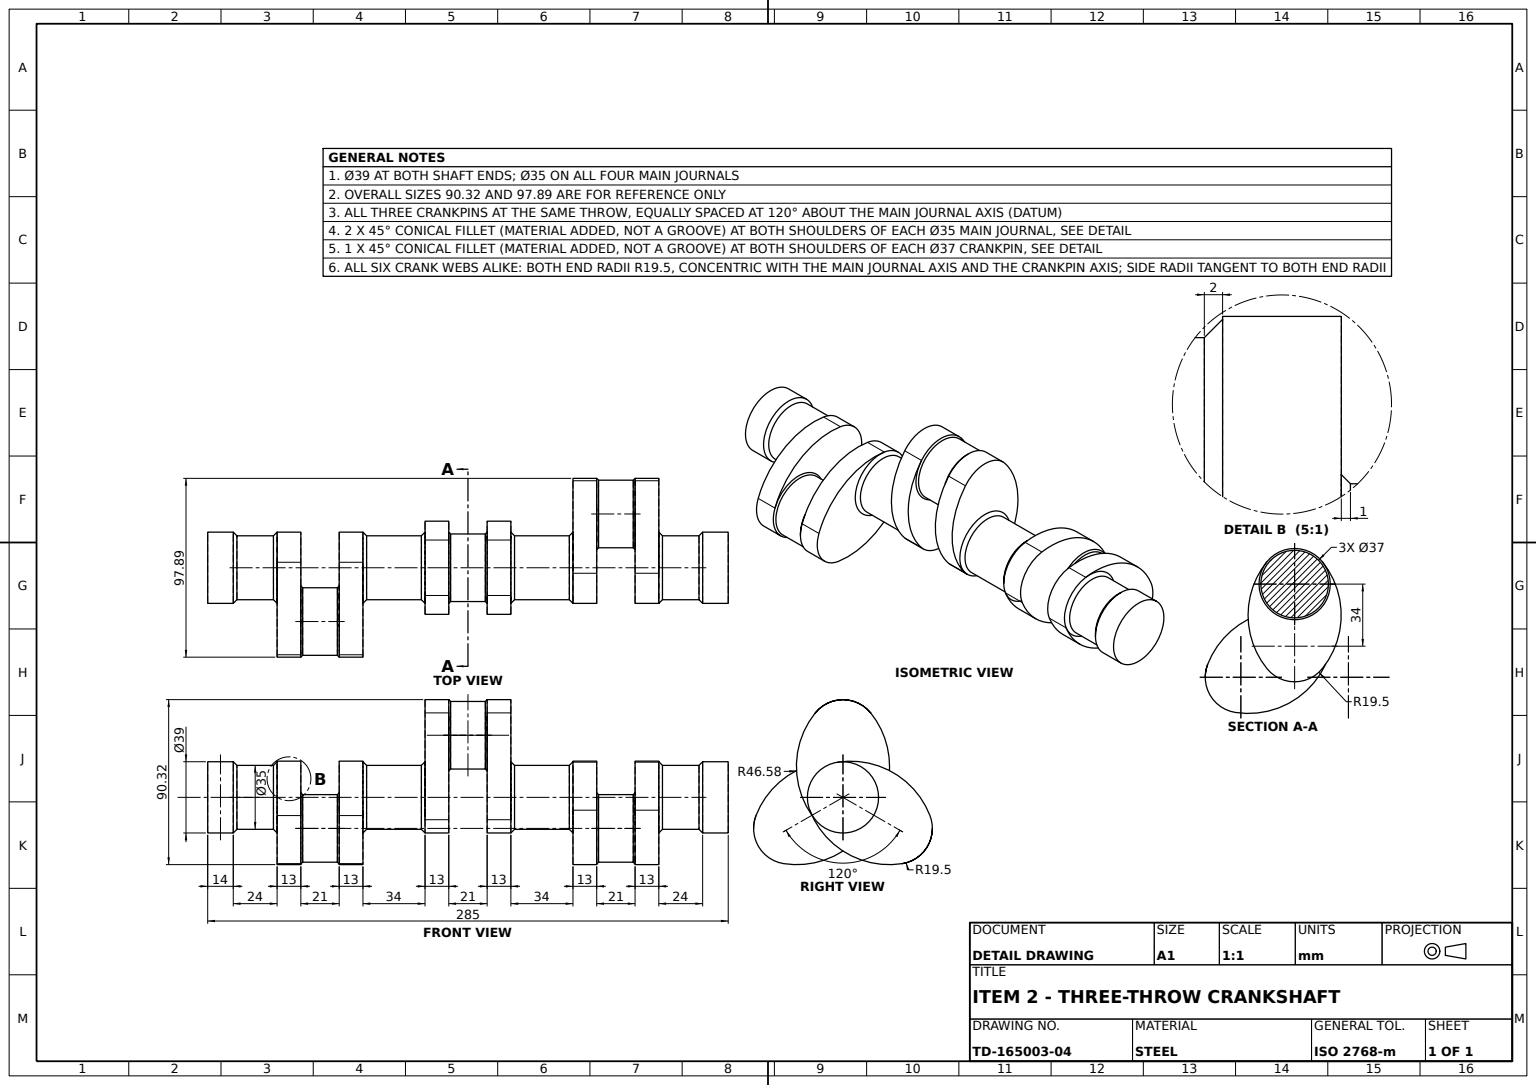
solid
v1 (247,0,19.5)
v2 (233,0,19.5)
e1 v1 v2 LINE
v3 (233,0,-19.5)
e2 v2 v3 CIRCLE(AX(P(233,0,0),D(1,0,0),D(0,0,-1)),19.5)
v4 (247,0,-19.5)
e3 v4 v3 LINE
e4 v1 v4 CIRCLE(AX(P(247,0,0),D(1,0,0),D(0,0,-1)),19.5)
face CYL(AX(P(247,0,0),D(-1,0,0),D(0,0,1)),19.5) [e1 e2 -e3 -e4]
v5 (196,-17,-9.9448637287)
v6 (196,-36.2662656294,-32.455014671)
e5 v5 v6 CIRCLE(AX(P(196,-17,-29.4448637287),D(1,0,0),D(0,0,1)),19.5)
v7 (196,-7.0262656294,18.1901509423)
e6 v7 v6 CIRCLE(AX(P(196,9.7587022631,-25.264098531),D(1,0,0),D(0,0,-1)),46.5833333333)
v8 (196,19.2662656294,3.0101509423)
e7 v8 v7 CIRCLE(AX(P(196,0,0),D(1,0,0),D(0,0,-1)),19.5)
v9 (196,-9.9737343706,-47.635014671)
e8 v9 v8 CIRCLE(AX(P(196,-26.7587022631,-4.1807651977),D(1,0,0),D(0,0,-1)),46.5833333333)
e9 v9 v5 CIRCLE(AX(P(196,-17,-29.4448637287),D(1,0,0),D(0,0,1)),19.5)
face PLANE(AX(P(196,-13.3793511316,-2.0903825988),D(-1,0,0),D(0,0,-1))) [e5 -e6 -e7 -e8 e9]
v10 (231,0,17.5)
e10 v10 v2 LINE
v11 (231,0,-17.5)
e11 v11 v10 CIRCLE(AX(P(231,0,0),D(-1,0,0),D(0,0,-1)),17.5)
e12 v11 v3 LINE
face CONE(AX(P(233,0,0),D(1,0,0),D(0,0,-1)),19.5,0.7853981634) [-e10 -e11 e12 -e2]
v12 (0,-9.9737343706,47.635014671)
v13 (0,-17,48.9448637287)
e13 v12 v13 CIRCLE(AX(P(0,-17,29.4448637287),D(1,0,0),D(0,0,-1)),19.5)
v14 (13,-17,48.9448637287)
e14 v14 v13 LINE
v15 (13,-9.9737343706,47.635014671)
e15 v15 v14 CIRCLE(AX(P(13,-17,29.4448637287),D(1,0,0),D(0,0,-1)),19.5)
e16 v15 v12 LINE
face CYL(AX(P(13,-17,29.4448637287),D(-1,0,0),D(0,0,1)),19.5) [e13 -e14 -e15 e16]
v16 (-38,0,19.5)
v17 (-38,0,-19.5)
e17 v16 v17 CIRCLE(AX(P(-38,0,0),D(1,0,0),D(0,0,-1)),19.5)
e18 v17 v16 CIRCLE(AX(P(-38,0,0),D(1,0,0),D(0,0,-1)),19.5)
face PLANE(AX(P(-38,19.5,0),D(-1,0,0),D(0,0,1))) [-e17 -e18]
v18 (-2,0,-17.5)
v19 (-2,0,17.5)
e19 v18 v19 CIRCLE(AX(P(-2,0,0),D(-1,0,0),D(0,0,1)),17.5)
v20 (0,0,-19.5)
e20 v18 v20 LINE
v21 (0,-7.0262656294,-18.1901509423)
e21 v21 v20 CIRCLE(AX(P(0,0,0),D(1,0,0),D(0,0,-1)),19.5)
v22 (0,0,19.5)
e22 v22 v21 CIRCLE(AX(P(0,0,0),D(1,0,0),D(0,0,1)),19.5)
e23 v19 v22 LINE
face CONE(AX(P(0,0,0),D(1,0,0),D(0,0,-1)),19.5,0.7853981634) [-e19 e20 -e21 -e22 -e23]
e24 v4 v1 CIRCLE(AX(P(247,0,0),D(1,0,0),D(0,0,-1)),19.5)
face PLANE(AX(P(247,0,0),D(1,0,0),D(0,0,-1))) [e24 e4]
v23 (128,-12.24,15.18)
v24 (128,-12.24,-15.18)
e25 v23 v24 CIRCLE(AX(P(128,0,0),D(1,0,0),D(0,0,-1)),19.5)
v25 (115,-12.24,15.18)
e26 v25 v23 LINE
v26 (115,-12.24,-15.18)
e27 v25 v26 CIRCLE(AX(P(115,0,0),D(1,0,0),D(0,0,-1)),19.5)
e28 v26 v24 LINE
face CYL(AX(P(115,0,0),D(1,0,0),D(0,0,-1)),19.5) [-e25 -e26 e27 e28]
v27 (114,34,18.5)
v28 (95,34,18.5)
e29 v27 v28 LINE
v29 (114,34,-18.5)
e30 v27 v29 CIRCLE(AX(P(114,34,0),D(-1,0,0),D(0,0,1)),18.5)
v30 (95,34,-18.5)
e31 v29 v30 LINE
e32 v30 v28 CIRCLE(AX(P(95,34,0),D(1,0,0),D(0,0,-1)),18.5)
face CYL(AX(P(115,34,0),D(-1,0,0),D(0,0,1)),18.5) [-e29 e30 e31 e32]
v31 (128,46.24,15.18)
e33 v31 v23 CIRCLE(AX(P(128,17,-21.0833333333),D(1,0,0),D(0,0,-1)),46.5833333333)
v32 (115,46.24,15.18)
e34 v32 v31 LINE
e35 v32 v25 CIRCLE(AX(P(115,17,-21.0833333333),D(1,0,0),D(0,0,-1)),46.5833333333)
face CYL(AX(P(115,17,-21.0833333333),D(1,0,0),D(0,0,-1)),46.5833333333) [e26 -e33 -e34 e35]
v33 (160,0,-17.5)
v34 (162,0,-19.5)
e36 v33 v34 LINE
v35 (162,-7.0262656294,18.1901509423)
e37 v35 v34 CIRCLE(AX(P(162,0,0),D(1,0,0),D(0,0,-1)),19.5)
v36 (162,0,19.5)
e38 v36 v35 CIRCLE(AX(P(162,0,0),D(1,0,0),D(0,0,-1)),19.5)
v37 (160,0,17.5)
e39 v37 v36 LINE
e40 v33 v37 CIRCLE(AX(P(160,0,0),D(-1,0,0),D(0,0,-1)),17.5)
face CONE(AX(P(162,0,0),D(1,0,0),D(0,0,-1)),19.5,0.7853981634) [e36 -e37 -e38 -e39 -e40]
v38 (49,0,-17.5)
v39 (49,0,17.5)
e41 v38 v39 CIRCLE(AX(P(49,0,0),D(1,0,0),D(0,0,-1)),17.5)
v40 (47,0,-19.5)
e42 v38 v40 LINE
v41 (47,19.2662656294,-3.0101509423)
e43 v40 v41 CIRCLE(AX(P(47,0,0),D(1,0,0),D(0,0,-1)),19.5)
v42 (47,0,19.5)
e44 v42 v41 CIRCLE(AX(P(47,0,0),D(-1,0,0),D(0,0,-1)),19.5)
e45 v39 v42 LINE
face CONE(AX(P(49,0,0),D(-1,0,0),D(0,0,1)),17.5,0.7853981634) [-e41 e42 e43 -e44 -e45]
v43 (195,-17,-47.9448637287)
v44 (176,-17,-47.9448637287)
e46 v43 v44 LINE
v45 (176,-17,-10.9448637287)
e47 v44 v45 CIRCLE(AX(P(176,-17,-29.4448637287),D(1,0,0),D(0,0,-1)),18.5)
v46 (195,-17,-10.9448637287)
e48 v46 v45 LINE
e49 v46 v43 CIRCLE(AX(P(195,-17,-29.4448637287),D(-1,0,0),D(0,0,1)),18.5)
face CYL(AX(P(196,-17,-29.4448637287),D(-1,0,0),D(0,0,1)),18.5) [e46 e47 -e48 e49]
e50 v37 v33 CIRCLE(AX(P(160,0,0),D(-1,0,0),D(0,0,-1)),17.5)
v47 (130,0,-17.5)
e51 v33 v47 LINE
v48 (130,0,17.5)
e52 v47 v48 CIRCLE(AX(P(130,0,0),D(1,0,0),D(0,0,1)),17.5)
e53 v37 v48 LINE
face CYL(AX(P(162,0,0),D(-1,0,0),D(0,0,1)),17.5) [e50 e51 e52 -e53]
v49 (33,-17,10.9448637287)
v50 (33,-17,47.9448637287)
e54 v49 v50 CIRCLE(AX(P(33,-17,29.4448637287),D(-1,0,0),D(0,0,-1)),18.5)
v51 (34,-17,9.9448637287)
e55 v49 v51 LINE
v52 (34,-36.2662656294,32.455014671)
e56 v52 v51 CIRCLE(AX(P(34,-17,29.4448637287),D(1,0,0),D(0,0,-1)),19.5)
v53 (34,-17,48.9448637287)
e57 v53 v52 CIRCLE(AX(P(34,-17,29.4448637287),D(1,0,0),D(0,0,-1)),19.5)
e58 v50 v53 LINE
face CONE(AX(P(34,-17,29.4448637287),D(1,0,0),D(0,0,-1)),19.5,0.7853981634) [-e54 e55 -e56 -e57 -e58]
v54 (94,46.24,-15.18)
v55 (94,46.24,15.18)
e59 v54 v55 CIRCLE(AX(P(94,34,0),D(1,0,0),D(0,0,-1)),19.5)
v56 (81,46.24,-15.18)
e60 v54 v56 LINE
v57 (81,46.24,15.18)
e61 v56 v57 CIRCLE(AX(P(81,34,0),D(1,0,0),D(0,0,-1)),19.5)
e62 v55 v57 LINE
face CYL(AX(P(94,34,0),D(-1,0,0),D(0,0,1)),19.5) [-e59 e60 e61 -e62]
e63 v10 v11 CIRCLE(AX(P(231,0,0),D(-1,0,0),D(0,0,-1)),17.5)
v58 (211,0,-17.5)
e64 v11 v58 LINE
v59 (211,0,17.5)
e65 v58 v59 CIRCLE(AX(P(211,0,0),D(1,0,0),D(0,0,1)),17.5)
e66 v10 v59 LINE
face CYL(AX(P(233,0,0),D(-1,0,0),D(0,0,1)),17.5) [e63 e64 e65 -e66]
v60 (34,-9.9737343706,47.635014671)
v61 (47,-9.9737343706,47.635014671)
e67 v60 v61 LINE
e68 v60 v53 CIRCLE(AX(P(34,-17,29.4448637287),D(1,0,0),D(0,0,-1)),19.5)
v62 (47,-36.2662656294,32.455014671)
e69 v52 v62 LINE
e70 v61 v62 CIRCLE(AX(P(47,-17,29.4448637287),D(1,0,0),D(0,0,-1)),19.5)
face CYL(AX(P(34,-17,29.4448637287),D(1,0,0),D(0,0,-1)),19.5) [-e67 e68 e57 e69 -e70]
e71 v29 v27 CIRCLE(AX(P(114,34,0),D(-1,0,0),D(0,0,1)),18.5)
e72 v28 v30 CIRCLE(AX(P(95,34,0),D(1,0,0),D(0,0,-1)),18.5)
face CYL(AX(P(115,34,0),D(-1,0,0),D(0,0,1)),18.5) [-e31 e71 e29 e72]
e73 v39 v38 CIRCLE(AX(P(49,0,0),D(1,0,0),D(0,0,-1)),17.5)
v63 (47,-7.0262656294,-18.1901509423)
e74 v63 v42 CIRCLE(AX(P(47,0,0),D(-1,0,0),D(0,0,-1)),19.5)
e75 v63 v40 CIRCLE(AX(P(47,0,0),D(1,0,0),D(0,0,-1)),19.5)
face CONE(AX(P(49,0,0),D(-1,0,0),D(0,0,1)),17.5,0.7853981634) [-e73 e45 -e74 e75 -e42]
v64 (13,-17,9.9448637287)
e76 v15 v64 CIRCLE(AX(P(13,-17,29.4448637287),D(-1,0,0),D(0,0,1)),19.5)
v65 (13,-36.2662656294,32.455014671)
e77 v64 v65 CIRCLE(AX(P(13,-17,29.4448637287),D(-1,0,0),D(0,0,1)),19.5)
v66 (13,-7.0262656294,-18.1901509423)
e78 v65 v66 CIRCLE(AX(P(13,9.7587022631,25.264098531),D(1,0,0),D(0,0,-1)),46.5833333333)
v67 (13,19.2662656294,-3.0101509423)
e79 v66 v67 CIRCLE(AX(P(13,0,0),D(1,0,0),D(0,0,-1)),19.5)
e80 v67 v15 CIRCLE(AX(P(13,-26.7587022631,4.1807651977),D(1,0,0),D(0,0,1)),46.5833333333)
face PLANE(AX(P(13,-13.3793511316,2.0903825988),D(-1,0,0),D(0,0,1))) rev [e76 e77 e78 e79 e80]
e81 v43 v46 CIRCLE(AX(P(195,-17,-29.4448637287),D(-1,0,0),D(0,0,1)),18.5)
e82 v45 v44 CIRCLE(AX(P(176,-17,-29.4448637287),D(1,0,0),D(0,0,-1)),18.5)
face CYL(AX(P(196,-17,-29.4448637287),D(-1,0,0),D(0,0,1)),18.5) [-e46 e81 e48 e82]
v68 (175,-9.9737343706,-47.635014671)
v69 (162,-9.9737343706,-47.635014671)
e83 v68 v69 LINE
v70 (175,-17,-48.9448637287)
e84 v70 v68 CIRCLE(AX(P(175,-17,-29.4448637287),D(1,0,0),D(0,0,-1)),19.5)
v71 (175,-36.2662656294,-32.455014671)
e85 v71 v70 CIRCLE(AX(P(175,-17,-29.4448637287),D(1,0,0),D(0,0,-1)),19.5)
v72 (162,-36.2662656294,-32.455014671)
e86 v71 v72 LINE
e87 v72 v69 CIRCLE(AX(P(162,-17,-29.4448637287),D(1,0,0),D(0,0,-1)),19.5)
face CYL(AX(P(175,-17,-29.4448637287),D(-1,0,0),D(0,0,1)),19.5) [-e83 -e84 -e85 e86 e87]
v73 (-24,0,-19.5)
e88 v17 v73 LINE
v74 (-24,0,19.5)
e89 v16 v74 LINE
e90 v73 v74 CIRCLE(AX(P(-24,0,0),D(1,0,0),D(0,0,-1)),19.5)
face CYL(AX(P(0,0,0),D(1,0,0),D(0,0,-1)),19.5) [-e88 e18 e89 -e90]
v75 (128,0,-19.5)
e91 v75 v24 CIRCLE(AX(P(128,0,0),D(-1,0,0),D(0,0,1)),19.5)
e92 v47 v75 LINE
e93 v48 v47 CIRCLE(AX(P(130,0,0),D(1,0,0),D(0,0,1)),17.5)
v76 (128,0,19.5)
e94 v48 v76 LINE
e95 v23 v76 CIRCLE(AX(P(128,0,0),D(-1,0,0),D(0,0,1)),19.5)
face CONE(AX(P(130,0,0),D(-1,0,0),D(0,0,1)),17.5,0.7853981634) [-e91 -e92 -e93 e94 -e95 e25]
e96 v3 v2 CIRCLE(AX(P(233,0,0),D(1,0,0),D(0,0,-1)),19.5)
face CYL(AX(P(247,0,0),D(-1,0,0),D(0,0,1)),19.5) [-e1 -e24 e3 e96]
v77 (79,0,-17.5)
e97 v77 v38 LINE
v78 (79,0,17.5)
e98 v78 v39 LINE
e99 v78 v77 CIRCLE(AX(P(79,0,0),D(-1,0,0),D(0,0,-1)),17.5)
face CYL(AX(P(81,0,0),D(-1,0,0),D(0,0,1)),17.5) [e97 e41 -e98 e99]
v79 (196,-17,-48.9448637287)
e100 v79 v9 CIRCLE(AX(P(196,-17,-29.4448637287),D(1,0,0),D(0,0,-1)),19.5)
e101 v43 v79 LINE
e102 v46 v5 LINE
face CONE(AX(P(196,-17,-29.4448637287),D(1,0,0),D(0,0,-1)),19.5,0.7853981634) [-e9 -e100 -e101 -e49 e102]
v80 (-22,0,17.5)
v81 (-22,0,-17.5)
e103 v80 v81 CIRCLE(AX(P(-22,0,0),D(1,0,0),D(0,0,-1)),17.5)
e104 v81 v18 LINE
e105 v80 v19 LINE
face CYL(AX(P(0,0,0),D(1,0,0),D(0,0,-1)),17.5) [e103 e104 e19 -e105]
v82 (162,19.2662656294,3.0101509423)
e106 v34 v82 CIRCLE(AX(P(162,0,0),D(1,0,0),D(0,0,-1)),19.5)
e107 v82 v36 CIRCLE(AX(P(162,0,0),D(1,0,0),D(0,0,-1)),19.5)
face CONE(AX(P(162,0,0),D(1,0,0),D(0,0,-1)),19.5,0.7853981634) [-e106 -e36 -e50 e39 -e107]
e108 v41 v61 CIRCLE(AX(P(47,-26.7587022631,4.1807651977),D(1,0,0),D(0,0,1)),46.5833333333)
e109 v62 v63 CIRCLE(AX(P(47,9.7587022631,25.264098531),D(1,0,0),D(0,0,-1)),46.5833333333)
face PLANE(AX(P(47,-13.3793511316,2.0903825988),D(1,0,0),D(0,0,1))) [e74 e44 e108 e70 e109]
e110 v59 v58 CIRCLE(AX(P(211,0,0),D(1,0,0),D(0,0,1)),17.5)
face CYL(AX(P(233,0,0),D(-1,0,0),D(0,0,1)),17.5) [-e64 e11 e66 e110]
e111 v80 v74 LINE
e112 v81 v80 CIRCLE(AX(P(-22,0,0),D(1,0,0),D(0,0,-1)),17.5)
e113 v81 v73 LINE
face CONE(AX(P(-22,0,0),D(-1,0,0),D(0,0,1)),17.5,0.7853981634) [e90 -e111 -e112 e113]
e114 v6 v79 CIRCLE(AX(P(196,-17,-29.4448637287),D(1,0,0),D(0,0,-1)),19.5)
face CONE(AX(P(196,-17,-29.4448637287),D(1,0,0),D(0,0,-1)),19.5,0.7853981634) [e101 -e114 -e5 -e102 -e81]
v83 (34,-7.0262656294,-18.1901509423)
e115 v83 v63 LINE
v84 (34,0,-19.5)
e116 v83 v84 CIRCLE(AX(P(34,0,0),D(1,0,0),D(0,0,-1)),19.5)
e117 v84 v40 LINE
face CYL(AX(P(34,0,0),D(1,0,0),D(0,0,-1)),19.5) [-e75 -e115 e116 e117]
v85 (81,0,19.5)
e118 v78 v85 LINE
v86 (81,0,-19.5)
e119 v86 v85 CIRCLE(AX(P(81,0,0),D(1,0,0),D(0,0,-1)),19.5)
e120 v77 v86 LINE
face CONE(AX(P(81,0,0),D(1,0,0),D(0,0,-1)),19.5,0.7853981634) [e118 -e119 -e120 -e99]
v87 (94,34,-19.5)
v88 (94,34,19.5)
e121 v87 v88 CIRCLE(AX(P(94,34,0),D(-1,0,0),D(0,0,-1)),19.5)
e122 v30 v87 LINE
e123 v28 v88 LINE
face CONE(AX(P(95,34,0),D(-1,0,0),D(0,0,1)),18.5,0.7853981634) [-e121 -e122 -e72 e123]
v89 (94,-12.24,15.18)
v90 (94,-12.24,-15.18)
e124 v89 v90 CIRCLE(AX(P(94,0,0),D(1,0,0),D(0,0,-1)),19.5)
v91 (81,-12.24,15.18)
e125 v89 v91 LINE
v92 (81,-12.24,-15.18)
e126 v91 v92 CIRCLE(AX(P(81,0,0),D(1,0,0),D(0,0,-1)),19.5)
e127 v90 v92 LINE
face CYL(AX(P(94,0,0),D(-1,0,0),D(0,0,1)),19.5) [-e124 e125 e126 -e127]
v93 (209,-7.0262656294,18.1901509423)
v94 (209,-36.2662656294,-32.455014671)
e128 v93 v94 CIRCLE(AX(P(209,9.7587022631,-25.264098531),D(1,0,0),D(0,0,-1)),46.5833333333)
v95 (209,-17,-48.9448637287)
e129 v94 v95 CIRCLE(AX(P(209,-17,-29.4448637287),D(1,0,0),D(0,0,-1)),19.5)
v96 (209,-9.9737343706,-47.635014671)
e130 v95 v96 CIRCLE(AX(P(209,-17,-29.4448637287),D(1,0,0),D(0,0,-1)),19.5)
v97 (209,19.2662656294,3.0101509423)
e131 v96 v97 CIRCLE(AX(P(209,-26.7587022631,-4.1807651977),D(1,0,0),D(0,0,-1)),46.5833333333)
v98 (209,0,-19.5)
e132 v97 v98 CIRCLE(AX(P(209,0,0),D(-1,0,0),D(0,0,1)),19.5)
e133 v98 v93 CIRCLE(AX(P(209,0,0),D(-1,0,0),D(0,0,1)),19.5)
face PLANE(AX(P(209,-13.3793511316,-2.0903825988),D(-1,0,0),D(0,0,-1))) rev [e128 e129 e130 e131 e132 e133]
v99 (0,-36.2662656294,32.455014671)
e134 v13 v99 CIRCLE(AX(P(0,-17,29.4448637287),D(1,0,0),D(0,0,-1)),19.5)
v100 (0,19.2662656294,-3.0101509423)
e135 v100 v12 CIRCLE(AX(P(0,-26.7587022631,4.1807651977),D(1,0,0),D(0,0,1)),46.5833333333)
e136 v100 v22 CIRCLE(AX(P(0,0,0),D(1,0,0),D(0,0,1)),19.5)
e137 v99 v21 CIRCLE(AX(P(0,9.7587022631,25.264098531),D(1,0,0),D(0,0,-1)),46.5833333333)
face PLANE(AX(P(0,-13.3793511316,2.0903825988),D(-1,0,0),D(0,0,1))) [-e134 -e13 -e135 e136 e22 -e137]
face CONE(AX(P(233,0,0),D(1,0,0),D(0,0,-1)),19.5,0.7853981634) [-e12 -e63 e10 -e96]
e138 v92 v56 CIRCLE(AX(P(81,17,21.0833333333),D(1,0,0),D(0,0,-1)),46.5833333333)
e139 v90 v54 CIRCLE(AX(P(94,17,21.0833333333),D(1,0,0),D(0,0,-1)),46.5833333333)
face CYL(AX(P(94,17,21.0833333333),D(-1,0,0),D(0,0,1)),46.5833333333) [e127 e138 -e60 -e139]
e140 v67 v100 LINE
face CYL(AX(P(13,-26.7587022631,4.1807651977),D(-1,0,0),D(0,0,1)),46.5833333333) [e135 -e16 -e80 e140]
e141 v9 v96 LINE
e142 v8 v97 LINE
face CYL(AX(P(196,-26.7587022631,-4.1807651977),D(1,0,0),D(0,0,-1)),46.5833333333) [-e131 -e141 e8 e142]
v101 (209,0,19.5)
e143 v101 v93 CIRCLE(AX(P(209,0,0),D(1,0,0),D(0,0,-1)),19.5)
e144 v58 v98 LINE
e145 v59 v101 LINE
face CONE(AX(P(211,0,0),D(-1,0,0),D(0,0,1)),17.5,0.7853981634) [e143 -e133 -e144 -e110 e145]
e146 v52 v83 CIRCLE(AX(P(34,9.7587022631,25.264098531),D(1,0,0),D(0,0,-1)),46.5833333333)
face CYL(AX(P(34,9.7587022631,25.264098531),D(1,0,0),D(0,0,-1)),46.5833333333) [e115 -e109 -e69 e146]
e147 v74 v73 CIRCLE(AX(P(-24,0,0),D(1,0,0),D(0,0,-1)),19.5)
face CONE(AX(P(-22,0,0),D(-1,0,0),D(0,0,1)),17.5,0.7853981634) [-e103 e111 e147 -e113]
v102 (115,34,-19.5)
e148 v29 v102 LINE
v103 (115,34,19.5)
e149 v103 v102 CIRCLE(AX(P(115,34,0),D(1,0,0),D(0,0,1)),19.5)
e150 v27 v103 LINE
face CONE(AX(P(115,34,0),D(1,0,0),D(0,0,-1)),19.5,0.7853981634) [-e71 e148 -e149 -e150]
e151 v97 v101 CIRCLE(AX(P(209,0,0),D(1,0,0),D(0,0,-1)),19.5)
face CONE(AX(P(211,0,0),D(-1,0,0),D(0,0,1)),17.5,0.7853981634) [e144 -e132 e151 -e145 -e65]
v104 (175,19.2662656294,3.0101509423)
e152 v68 v104 CIRCLE(AX(P(175,-26.7587022631,-4.1807651977),D(1,0,0),D(0,0,-1)),46.5833333333)
e153 v69 v82 CIRCLE(AX(P(162,-26.7587022631,-4.1807651977),D(1,0,0),D(0,0,-1)),46.5833333333)
e154 v104 v82 LINE
face CYL(AX(P(175,-26.7587022631,-4.1807651977),D(-1,0,0),D(0,0,1)),46.5833333333) [-e152 e83 e153 -e154]
e155 v92 v86 CIRCLE(AX(P(81,0,0),D(1,0,0),D(0,0,-1)),19.5)
e156 v85 v91 CIRCLE(AX(P(81,0,0),D(1,0,0),D(0,0,-1)),19.5)
e157 v77 v78 CIRCLE(AX(P(79,0,0),D(-1,0,0),D(0,0,-1)),17.5)
face CONE(AX(P(81,0,0),D(1,0,0),D(0,0,-1)),19.5,0.7853981634) [e120 -e155 -e126 -e156 -e118 -e157]
e158 v6 v94 LINE
e159 v7 v93 LINE
face CYL(AX(P(196,9.7587022631,-25.264098531),D(1,0,0),D(0,0,-1)),46.5833333333) [e6 e158 -e128 -e159]
v105 (14,-17,10.9448637287)
e160 v49 v105 LINE
v106 (14,-17,47.9448637287)
e161 v105 v106 CIRCLE(AX(P(14,-17,29.4448637287),D(1,0,0),D(0,0,1)),18.5)
e162 v50 v106 LINE
e163 v50 v49 CIRCLE(AX(P(33,-17,29.4448637287),D(-1,0,0),D(0,0,-1)),18.5)
face CYL(AX(P(34,-17,29.4448637287),D(-1,0,0),D(0,0,1)),18.5) [e160 e161 -e162 e163]
e164 v79 v95 LINE
face CYL(AX(P(196,-17,-29.4448637287),D(1,0,0),D(0,0,-1)),19.5) [-e164 e100 e141 -e130]
v107 (175,0,19.5)
e165 v107 v36 LINE
e166 v104 v107 CIRCLE(AX(P(175,0,0),D(1,0,0),D(0,0,-1)),19.5)
face CYL(AX(P(175,0,0),D(-1,0,0),D(0,0,1)),19.5) [e107 -e165 -e166 e154]
e167 v35 v72 CIRCLE(AX(P(162,9.7587022631,-25.264098531),D(1,0,0),D(0,0,-1)),46.5833333333)
face PLANE(AX(P(162,-13.3793511316,-2.0903825988),D(1,0,0),D(0,0,-1))) rev [e106 -e153 -e87 -e167 e37]
e168 v76 v75 CIRCLE(AX(P(128,0,0),D(-1,0,0),D(0,0,1)),19.5)
face CONE(AX(P(130,0,0),D(-1,0,0),D(0,0,1)),17.5,0.7853981634) [e92 -e168 -e94 -e52]
v108 (128,17,-25.5)
e169 v24 v108 CIRCLE(AX(P(128,17,21.0833333333),D(1,0,0),D(0,0,-1)),46.5833333333)
v109 (115,17,-25.5)
e170 v26 v109 CIRCLE(AX(P(115,17,21.0833333333),D(1,0,0),D(0,0,-1)),46.5833333333)
e171 v109 v108 LINE
face CYL(AX(P(115,17,21.0833333333),D(1,0,0),D(0,0,-1)),46.5833333333) [-e169 -e28 e170 e171]
v110 (175,-7.0262656294,18.1901509423)
e172 v107 v110 CIRCLE(AX(P(175,0,0),D(1,0,0),D(0,0,-1)),19.5)
e173 v110 v35 LINE
face CYL(AX(P(175,0,0),D(-1,0,0),D(0,0,1)),19.5) [-e172 e165 e38 -e173]
v111 (34,19.2662656294,-3.0101509423)
e174 v84 v111 CIRCLE(AX(P(34,0,0),D(1,0,0),D(0,0,-1)),19.5)
e175 v111 v41 LINE
face CYL(AX(P(34,0,0),D(1,0,0),D(0,0,-1)),19.5) [-e43 -e117 e174 e175]
e176 v51 v60 CIRCLE(AX(P(34,-17,29.4448637287),D(1,0,0),D(0,0,-1)),19.5)
e177 v111 v60 CIRCLE(AX(P(34,-26.7587022631,4.1807651977),D(1,0,0),D(0,0,1)),46.5833333333)
face PLANE(AX(P(34,-13.3793511316,2.0903825988),D(1,0,0),D(0,0,1))) rev [e176 -e177 -e174 -e116 -e146 e56]
v112 (115,46.24,-15.18)
e178 v109 v112 CIRCLE(AX(P(115,17,21.0833333333),D(1,0,0),D(0,0,-1)),46.5833333333)
v113 (128,46.24,-15.18)
e179 v112 v113 LINE
e180 v108 v113 CIRCLE(AX(P(128,17,21.0833333333),D(1,0,0),D(0,0,-1)),46.5833333333)
face CYL(AX(P(115,17,21.0833333333),D(1,0,0),D(0,0,-1)),46.5833333333) [-e171 e178 e179 -e180]
e181 v44 v70 LINE
v114 (175,-17,-9.9448637287)
e182 v45 v114 LINE
e183 v71 v114 CIRCLE(AX(P(175,-17,-29.4448637287),D(-1,0,0),D(0,0,-1)),19.5)
face CONE(AX(P(176,-17,-29.4448637287),D(-1,0,0),D(0,0,1)),18.5,0.7853981634) [e85 -e181 -e82 e182 -e183]
e184 v114 v68 CIRCLE(AX(P(175,-17,-29.4448637287),D(-1,0,0),D(0,0,-1)),19.5)
face CONE(AX(P(176,-17,-29.4448637287),D(-1,0,0),D(0,0,1)),18.5,0.7853981634) [e84 -e184 -e182 -e47 e181]
e185 v106 v105 CIRCLE(AX(P(14,-17,29.4448637287),D(1,0,0),D(0,0,1)),18.5)
face CYL(AX(P(34,-17,29.4448637287),D(-1,0,0),D(0,0,1)),18.5) [e54 e162 e185 -e160]
e186 v32 v103 CIRCLE(AX(P(115,34,0),D(1,0,0),D(0,0,1)),19.5)
e187 v102 v112 CIRCLE(AX(P(115,34,0),D(1,0,0),D(0,0,1)),19.5)
face PLANE(AX(P(115,8.5,-10.5416666667),D(-1,0,0),D(0,0,-1))) [-e170 -e27 -e35 e186 e149 e187 -e178]
e188 v19 v18 CIRCLE(AX(P(-2,0,0),D(-1,0,0),D(0,0,1)),17.5)
face CYL(AX(P(0,0,0),D(1,0,0),D(0,0,-1)),17.5) [e188 -e104 e112 e105]
face CYL(AX(P(0,0,0),D(1,0,0),D(0,0,-1)),19.5) [e17 e88 -e147 -e89]
e189 v14 v65 CIRCLE(AX(P(13,-17,29.4448637287),D(1,0,0),D(0,0,-1)),19.5)
e190 v65 v99 LINE
face CYL(AX(P(13,-17,29.4448637287),D(-1,0,0),D(0,0,1)),19.5) [-e189 e14 e134 -e190]
e191 v66 v21 LINE
face CYL(AX(P(13,9.7587022631,25.264098531),D(-1,0,0),D(0,0,1)),46.5833333333) [e137 -e191 -e78 e190]
e192 v105 v64 LINE
e193 v106 v14 LINE
face CONE(AX(P(14,-17,29.4448637287),D(-1,0,0),D(0,0,1)),18.5,0.7853981634) [e189 -e77 -e192 -e185 e193]
v115 (94,17,25.5)
v116 (81,17,25.5)
e194 v115 v116 LINE
e195 v116 v91 CIRCLE(AX(P(81,17,-21.0833333333),D(1,0,0),D(0,0,-1)),46.5833333333)
e196 v115 v89 CIRCLE(AX(P(94,17,-21.0833333333),D(1,0,0),D(0,0,-1)),46.5833333333)
face CYL(AX(P(94,17,-21.0833333333),D(-1,0,0),D(0,0,1)),46.5833333333) [e194 e195 -e125 -e196]
face CYL(AX(P(196,0,0),D(1,0,0),D(0,0,-1)),19.5) [-e143 -e151 -e142 e7 e159]
face CYL(AX(P(81,0,0),D(-1,0,0),D(0,0,1)),17.5) [e98 e73 -e97 e157]
face CONE(AX(P(34,-17,29.4448637287),D(1,0,0),D(0,0,-1)),19.5,0.7853981634) [e58 -e68 -e176 -e55 -e163]
e197 v110 v71 CIRCLE(AX(P(175,9.7587022631,-25.264098531),D(1,0,0),D(0,0,-1)),46.5833333333)
face PLANE(AX(P(175,-13.3793511316,-2.0903825988),D(1,0,0),D(0,0,-1))) [e197 e183 e184 e152 e166 e172]
e198 v88 v55 CIRCLE(AX(P(94,34,0),D(-1,0,0),D(0,0,-1)),19.5)
e199 v54 v87 CIRCLE(AX(P(94,34,0),D(-1,0,0),D(0,0,-1)),19.5)
face CONE(AX(P(95,34,0),D(-1,0,0),D(0,0,1)),18.5,0.7853981634) [e59 -e198 -e123 -e32 e122 -e199]
e200 v55 v115 CIRCLE(AX(P(94,17,-21.0833333333),D(1,0,0),D(0,0,-1)),46.5833333333)
e201 v57 v116 CIRCLE(AX(P(81,17,-21.0833333333),D(1,0,0),D(0,0,-1)),46.5833333333)
face CYL(AX(P(94,17,-21.0833333333),D(-1,0,0),D(0,0,1)),46.5833333333) [-e194 -e200 e62 e201]
e202 v113 v31 CIRCLE(AX(P(128,34,0),D(1,0,0),D(0,0,-1)),19.5)
face PLANE(AX(P(128,8.5,-10.5416666667),D(-1,0,0),D(0,0,-1))) rev [e95 e168 e91 e169 e180 e202 e33]
e203 v20 v100 CIRCLE(AX(P(0,0,0),D(1,0,0),D(0,0,-1)),19.5)
face CYL(AX(P(13,0,0),D(-1,0,0),D(0,0,1)),19.5) [e203 -e140 -e79 e191 e21]
face CYL(AX(P(175,9.7587022631,-25.264098531),D(-1,0,0),D(0,0,1)),46.5833333333) [e167 -e86 -e197 e173]
face PLANE(AX(P(81,8.5,-10.5416666667),D(1,0,0),D(0,0,-1))) rev [e119 e156 -e195 -e201 -e61 -e138 e155]
face CONE(AX(P(0,0,0),D(1,0,0),D(0,0,-1)),19.5,0.7853981634) [e23 -e136 -e203 -e20 -e188]
face CYL(AX(P(196,-17,-29.4448637287),D(1,0,0),D(0,0,-1)),19.5) [-e129 -e158 e114 e164]
e204 v112 v32 CIRCLE(AX(P(115,34,0),D(1,0,0),D(0,0,-1)),19.5)
face CONE(AX(P(115,34,0),D(1,0,0),D(0,0,-1)),19.5,0.7853981634) [-e204 -e187 -e148 -e30 e150 -e186]
face CONE(AX(P(14,-17,29.4448637287),D(-1,0,0),D(0,0,1)),18.5,0.7853981634) [e192 -e76 e15 -e193 -e161]
face PLANE(AX(P(94,8.5,-10.5416666667),D(1,0,0),D(0,0,-1))) [e139 e199 e121 e198 e200 e196 e124]
face CYL(AX(P(115,34,0),D(1,0,0),D(0,0,-1)),19.5) [e204 e34 -e202 -e179]
face CYL(AX(P(162,0,0),D(-1,0,0),D(0,0,1)),17.5) [e40 e53 e93 -e51]
face CYL(AX(P(34,-26.7587022631,4.1807651977),D(1,0,0),D(0,0,-1)),46.5833333333) [-e108 -e175 e177 e67]
